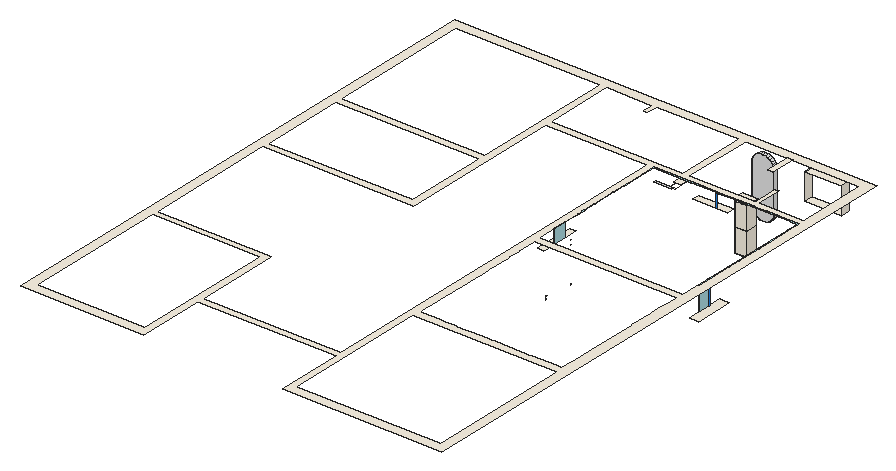
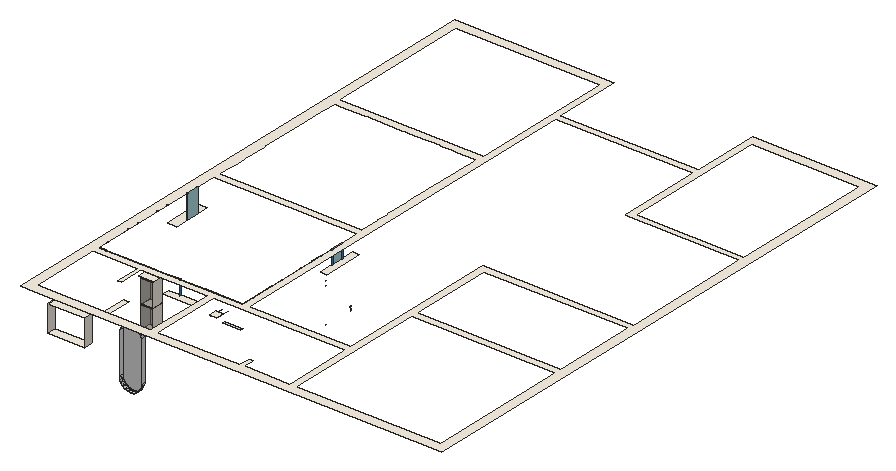
# SketchUp Ruby script. Lengths in inches.
U = 1.inch
M = Sketchup.active_model
def pt(a) = Geom::Point3d.new(a.map { |v| v * U })
def face(e, loops, mat)
  f = e.add_face(loops[0].map { |a| pt(a) })
  loops[1..].each { |l| e.add_face(l.map { |a| pt(a) }).erase! }
  f.material = f.back_material = mat if mat
  f
end
# faces: each face lists its corners as indices into pts; further lists are holes
def faces(e, pts, list, mat = nil) = list.each { |f| face(e, (f[0].is_a?(Array) ? f : [f]).map { |l| l.map { |i| pts[i] } }, mat) }
# xy, xz, yz: faces in a plane at the given z, y or x. An outline is a flat list of corners, or four numbers for a rectangle; further outlines are holes
def ring(l) = l.size == 4 ? [[l[0], l[1]], [l[2], l[1]], [l[2], l[3]], [l[0], l[3]]] : l.each_slice(2).to_a
def flat(e, list, mat, &to3) = list.each { |f| face(e, (f[0].is_a?(Array) ? f : [f]).map { |l| ring(l).map { |u, v| to3.(u, v) } }, mat) }
def xy(e, z, list, mat = nil) = flat(e, list, mat) { |x, y| [x, y, z] }
def xz(e, y, list, mat = nil) = flat(e, list, mat) { |x, z| [x, y, z] }
def yz(e, x, list, mat = nil) = flat(e, list, mat) { |y, z| [x, y, z] }
def lines(e, pts, list) = list.each { |a, b| e.add_line(pt(pts[a]), pt(pts[b])) }
# prism: a flat outline (further loops are holes) pulled along v
def prism(e, loops, v, mat = nil)
  f = face(e, loops, mat); d = Geom::Vector3d.new(v.map { |x| x * U })
  f.pushpull(f.normal.samedirection?(d) ? d.length : -d.length)
end
def box(e, o, s, mat = nil) = prism(e, [[o, [o[0] + s[0], o[1], o[2]], [o[0] + s[0], o[1] + s[1], o[2]], [o[0], o[1] + s[1], o[2]]]], [0, 0, s[2]], mat)
def at(x, y, z, deg = 0) = Geom::Transformation.translation(pt([x, y, z])) * Geom::Transformation.rotation(ORIGIN, Z_AXIS, deg.degrees)
def axes(o, x, y, z) = Geom::Transformation.new([*x, 0, *y, 0, *z, 0, *pt(o).to_a, 1])
def part(name) = M.definitions.add(name)
# library, detail: a bought-in or finely detailed component or shape, given as its bounding box
def library(name, o, s) = part(name).tap { |d| box(d.entities, o, s) }
def detail(e, o, s) = box(e.add_group.entities, o, s)
def put(e, d, t, mat = nil) = e.add_instance(d, t).tap { |i| i.material = mat if mat }
def group(e, t, mat = nil) = e.add_group.tap { |g| g.transformation = t; g.material = mat if mat }.entities
root = M.entities
M.materials.add("Material \#1").color = [140, 140, 140]
M.materials.add("[0030_OldLace]").color = [253, 245, 230]
M.materials.add("[0094_PowderBlue]").color = [176, 224, 230]
M.materials.add("[0098_DodgerBlue]").color = [30, 144, 255]
M.materials.add("[Mirror 02]").color = [229, 229, 229]
M.materials.add("[Translucent Glass Gray]").color = [128, 128, 128]
M.materials["[Translucent Glass Gray]"].alpha = 0.5
xy(root,58.602,[[264.049,358.92,264.049,358.939,264.045,358.932],[264.049,358.92,264.053,358.949,264.049,358.939],[264.049,358.92,264.054,358.932,264.053,358.949],[264.045,358.932,264.046,358.949,264.041,358.964],[264.045,358.932,264.049,358.939,264.046,358.949],
  [264.054,358.932,264.057,358.978,264.053,358.949],[264.054,358.932,264.058,358.964,264.057,358.978],[264.046,358.949,264.042,358.978,264.041,358.964],[264.041,358.964,264.042,358.978,264.038,359.014],[264.058,358.964,264.059,359.023,264.057,358.978],
  [264.058,358.964,264.061,359.014,264.059,359.023],[264.042,358.978,264.039,359.023,264.038,359.014],[264.038,359.014,264.039,359.023,264.037,359.075],[264.061,359.014,264.061,359.078,264.059,359.023],[264.061,359.014,264.062,359.075,264.061,359.078],
  [264.039,359.023,264.038,359.078,264.037,359.075],[264.037,359.075,264.038,359.078,264.037,359.14],[264.062,359.075,264.061,359.137,264.061,359.078],[264.062,359.075,264.062,359.14,264.061,359.137],[264.038,359.078,264.038,359.137,264.037,359.14],
  [264.038,359.137,264.038,359.201,264.037,359.14],[264.038,359.137,264.039,359.192,264.038,359.201],[264.061,359.137,264.062,359.14,264.059,359.192],[264.062,359.14,264.061,359.201,264.059,359.192],[264.039,359.192,264.041,359.251,264.038,359.201],
  [264.039,359.192,264.042,359.237,264.041,359.251],[264.059,359.192,264.061,359.201,264.057,359.237],[264.061,359.201,264.058,359.251,264.057,359.237],[264.042,359.237,264.045,359.284,264.041,359.251],[264.042,359.237,264.046,359.266,264.045,359.284],
  [264.057,359.237,264.058,359.251,264.053,359.266],[264.058,359.251,264.054,359.284,264.053,359.266],[264.046,359.266,264.049,359.295,264.045,359.284],[264.046,359.266,264.049,359.276,264.049,359.295],[264.053,359.266,264.054,359.284,264.049,359.276],
  [264.049,359.276,264.054,359.284,264.049,359.295]],"Material \#1")
xy(root,58.622,[[264.049,358.92,264.045,358.932,264.046,358.949],[264.049,358.92,264.046,358.949,264.049,358.939],[264.049,358.92,264.049,358.939,264.054,358.932],[264.045,358.932,264.041,358.964,264.042,358.978],[264.045,358.932,264.042,358.978,264.046,358.949],
  [264.054,358.932,264.049,358.939,264.053,358.949],[264.054,358.932,264.053,358.949,264.058,358.964],[264.053,358.949,264.057,358.978,264.058,358.964],[264.041,358.964,264.038,359.014,264.039,359.023],[264.041,358.964,264.039,359.023,264.042,358.978],
  [264.058,358.964,264.057,358.978,264.061,359.014],[264.057,358.978,264.059,359.023,264.061,359.014],[264.038,359.014,264.037,359.075,264.038,359.078],[264.038,359.014,264.038,359.078,264.039,359.023],[264.061,359.014,264.059,359.023,264.062,359.075],
  [264.059,359.023,264.061,359.078,264.062,359.075],[264.037,359.075,264.037,359.14,264.038,359.137],[264.037,359.075,264.038,359.137,264.038,359.078],[264.062,359.075,264.061,359.078,264.062,359.14],[264.061,359.078,264.061,359.137,264.062,359.14],
  [264.038,359.137,264.037,359.14,264.039,359.192],[264.061,359.137,264.059,359.192,264.061,359.201],[264.061,359.137,264.061,359.201,264.062,359.14],[264.037,359.14,264.038,359.201,264.039,359.192],[264.039,359.192,264.038,359.201,264.042,359.237],
  [264.059,359.192,264.057,359.237,264.058,359.251],[264.059,359.192,264.058,359.251,264.061,359.201],[264.038,359.201,264.041,359.251,264.042,359.237],[264.042,359.237,264.041,359.251,264.046,359.266],[264.057,359.237,264.053,359.266,264.054,359.284],
  [264.057,359.237,264.054,359.284,264.058,359.251],[264.041,359.251,264.045,359.284,264.046,359.266],[264.046,359.266,264.045,359.284,264.049,359.276],[264.053,359.266,264.049,359.276,264.049,359.295],[264.053,359.266,264.049,359.295,264.054,359.284],
  [264.049,359.276,264.045,359.284,264.049,359.295]],"Material \#1")
xy(root,70.574,[[346.166,460.902,357.778,472.402]],"[0030_OldLace]")
xy(root,71.074,[[346.166,460.902,357.778,472.402]],"[0030_OldLace]")
xy(root,87.625,[[356.125,535.465,392.375,544.465]],"[0030_OldLace]")
xy(root,93.657,[[346.166,460.902,357.778,472.402]],"[0030_OldLace]")
xy(root,93.765,[[264.049,358.92,264.046,358.949,264.045,358.932],[264.049,358.92,264.049,358.939,264.046,358.949],[264.049,358.92,264.054,358.932,264.049,358.939],[264.045,358.932,264.042,358.978,264.041,358.964],[264.045,358.932,264.046,358.949,264.042,358.978],
  [264.054,358.932,264.053,358.949,264.049,358.939],[264.054,358.932,264.058,358.964,264.053,358.949],[264.053,358.949,264.058,358.964,264.057,358.978],[264.041,358.964,264.039,359.023,264.038,359.014],[264.041,358.964,264.042,358.978,264.039,359.023],
  [264.058,358.964,264.061,359.014,264.057,358.978],[264.057,358.978,264.061,359.014,264.059,359.023],[264.038,359.014,264.038,359.078,264.037,359.075],[264.038,359.014,264.039,359.023,264.038,359.078],[264.061,359.014,264.062,359.075,264.059,359.023],
  [264.059,359.023,264.062,359.075,264.061,359.078],[264.037,359.075,264.038,359.078,264.038,359.137],[264.037,359.075,264.038,359.137,264.037,359.14],[264.062,359.075,264.062,359.14,264.061,359.078],[264.061,359.078,264.062,359.14,264.061,359.137],
  [264.038,359.137,264.039,359.192,264.037,359.14],[264.061,359.137,264.061,359.201,264.059,359.192],[264.061,359.137,264.062,359.14,264.061,359.201],[264.037,359.14,264.039,359.192,264.038,359.201],[264.039,359.192,264.042,359.237,264.038,359.201],
  [264.059,359.192,264.058,359.251,264.057,359.237],[264.059,359.192,264.061,359.201,264.058,359.251],[264.038,359.201,264.042,359.237,264.041,359.251],[264.042,359.237,264.046,359.266,264.041,359.251],[264.057,359.237,264.054,359.284,264.053,359.266],
  [264.057,359.237,264.058,359.251,264.054,359.284],[264.041,359.251,264.046,359.266,264.045,359.284],[264.046,359.266,264.049,359.276,264.045,359.284],[264.053,359.266,264.049,359.295,264.049,359.276],[264.053,359.266,264.054,359.284,264.049,359.295],
  [264.049,359.276,264.049,359.295,264.045,359.284]],"Material \#1")
xy(root,93.785,[[264.049,358.92,264.045,358.932,264.049,358.939],[264.049,358.92,264.049,358.939,264.053,358.949],[264.049,358.92,264.053,358.949,264.054,358.932],[264.045,358.932,264.041,358.964,264.046,358.949],[264.045,358.932,264.046,358.949,264.049,358.939],
  [264.054,358.932,264.053,358.949,264.057,358.978],[264.054,358.932,264.057,358.978,264.058,358.964],[264.046,358.949,264.041,358.964,264.042,358.978],[264.041,358.964,264.038,359.014,264.042,358.978],[264.058,358.964,264.057,358.978,264.059,359.023],
  [264.058,358.964,264.059,359.023,264.061,359.014],[264.042,358.978,264.038,359.014,264.039,359.023],[264.038,359.014,264.037,359.075,264.039,359.023],[264.061,359.014,264.059,359.023,264.061,359.078],[264.061,359.014,264.061,359.078,264.062,359.075],
  [264.039,359.023,264.037,359.075,264.038,359.078],[264.037,359.075,264.037,359.14,264.038,359.078],[264.062,359.075,264.061,359.078,264.061,359.137],[264.062,359.075,264.061,359.137,264.062,359.14],[264.038,359.078,264.037,359.14,264.038,359.137],
  [264.038,359.137,264.037,359.14,264.038,359.201],[264.038,359.137,264.038,359.201,264.039,359.192],[264.061,359.137,264.059,359.192,264.062,359.14],[264.062,359.14,264.059,359.192,264.061,359.201],[264.039,359.192,264.038,359.201,264.041,359.251],
  [264.039,359.192,264.041,359.251,264.042,359.237],[264.059,359.192,264.057,359.237,264.061,359.201],[264.061,359.201,264.057,359.237,264.058,359.251],[264.042,359.237,264.041,359.251,264.045,359.284],[264.042,359.237,264.045,359.284,264.046,359.266],
  [264.057,359.237,264.053,359.266,264.058,359.251],[264.058,359.251,264.053,359.266,264.054,359.284],[264.046,359.266,264.045,359.284,264.049,359.295],[264.046,359.266,264.049,359.295,264.049,359.276],[264.053,359.266,264.049,359.276,264.054,359.284],
  [264.049,359.276,264.049,359.295,264.054,359.284]],"Material \#1")
xy(root,94.157,[[346.166,460.902,357.778,472.402]],"[0030_OldLace]")
xy(root,96,[[410.75,323.465,410.75,334.965,411,334.965,411,335.465,410.75,335.465,410.75,347.465,411,347.465,411,347.965,410.75,347.965,410.75,361.527,420,361.527,420,323.465]],"[0030_OldLace]")
xy(root,98.228,[[264.049,358.92,264.049,358.939,264.045,358.932],[264.049,358.92,264.053,358.949,264.049,358.939],[264.049,358.92,264.054,358.932,264.053,358.949],[264.045,358.932,264.046,358.949,264.041,358.964],[264.045,358.932,264.049,358.939,264.046,358.949],
  [264.054,358.932,264.057,358.978,264.053,358.949],[264.054,358.932,264.058,358.964,264.057,358.978],[264.046,358.949,264.042,358.978,264.041,358.964],[264.041,358.964,264.042,358.978,264.038,359.014],[264.058,358.964,264.059,359.023,264.057,358.978],
  [264.058,358.964,264.061,359.014,264.059,359.023],[264.042,358.978,264.039,359.023,264.038,359.014],[264.038,359.014,264.039,359.023,264.037,359.075],[264.061,359.014,264.061,359.078,264.059,359.023],[264.061,359.014,264.062,359.075,264.061,359.078],
  [264.039,359.023,264.038,359.078,264.037,359.075],[264.037,359.075,264.038,359.078,264.037,359.14],[264.062,359.075,264.061,359.137,264.061,359.078],[264.062,359.075,264.062,359.14,264.061,359.137],[264.038,359.078,264.038,359.137,264.037,359.14],
  [264.038,359.137,264.038,359.201,264.037,359.14],[264.038,359.137,264.039,359.192,264.038,359.201],[264.061,359.137,264.062,359.14,264.059,359.192],[264.062,359.14,264.061,359.201,264.059,359.192],[264.039,359.192,264.041,359.251,264.038,359.201],
  [264.039,359.192,264.042,359.237,264.041,359.251],[264.059,359.192,264.061,359.201,264.057,359.237],[264.061,359.201,264.058,359.251,264.057,359.237],[264.042,359.237,264.045,359.284,264.041,359.251],[264.042,359.237,264.046,359.266,264.045,359.284],
  [264.057,359.237,264.058,359.251,264.053,359.266],[264.058,359.251,264.054,359.284,264.053,359.266],[264.046,359.266,264.049,359.295,264.045,359.284],[264.046,359.266,264.049,359.276,264.049,359.295],[264.053,359.266,264.054,359.284,264.049,359.276],
  [264.049,359.276,264.054,359.284,264.049,359.295]],"Material \#1")
xy(root,98.248,[[264.049,358.92,264.045,358.932,264.046,358.949],[264.049,358.92,264.046,358.949,264.049,358.939],[264.049,358.92,264.049,358.939,264.054,358.932],[264.045,358.932,264.041,358.964,264.042,358.978],[264.045,358.932,264.042,358.978,264.046,358.949],
  [264.054,358.932,264.049,358.939,264.053,358.949],[264.054,358.932,264.053,358.949,264.058,358.964],[264.053,358.949,264.057,358.978,264.058,358.964],[264.041,358.964,264.038,359.014,264.039,359.023],[264.041,358.964,264.039,359.023,264.042,358.978],
  [264.058,358.964,264.057,358.978,264.061,359.014],[264.057,358.978,264.059,359.023,264.061,359.014],[264.038,359.014,264.037,359.075,264.038,359.078],[264.038,359.014,264.038,359.078,264.039,359.023],[264.061,359.014,264.059,359.023,264.062,359.075],
  [264.059,359.023,264.061,359.078,264.062,359.075],[264.037,359.075,264.037,359.14,264.038,359.137],[264.037,359.075,264.038,359.137,264.038,359.078],[264.062,359.075,264.061,359.078,264.062,359.14],[264.061,359.078,264.061,359.137,264.062,359.14],
  [264.038,359.137,264.037,359.14,264.039,359.192],[264.061,359.137,264.059,359.192,264.061,359.201],[264.061,359.137,264.061,359.201,264.062,359.14],[264.037,359.14,264.038,359.201,264.039,359.192],[264.039,359.192,264.038,359.201,264.042,359.237],
  [264.059,359.192,264.057,359.237,264.058,359.251],[264.059,359.192,264.058,359.251,264.061,359.201],[264.038,359.201,264.041,359.251,264.042,359.237],[264.042,359.237,264.041,359.251,264.046,359.266],[264.057,359.237,264.053,359.266,264.054,359.284],
  [264.057,359.237,264.054,359.284,264.058,359.251],[264.041,359.251,264.045,359.284,264.046,359.266],[264.046,359.266,264.045,359.284,264.049,359.276],[264.053,359.266,264.049,359.276,264.049,359.295],[264.053,359.266,264.049,359.295,264.054,359.284],
  [264.049,359.276,264.045,359.284,264.049,359.295]],"Material \#1")
xy(root,102.757,[[262.134,465.465,279.821,468.027]],"[Mirror 02]")
xy(root,106,[[261,321.882,261,361.777,267.4375,361.777,267.4375,347.965,267,347.965,267,347.465,267.4375,347.465,267.4375,335.465,267,335.465,267,334.965,267.4375,334.965,267.4375,321.882],[306.3125,458.34,306.3125,465.465,341.0625,465.465,341.0625,458.34,329.5,458.34,329.5,459.465,329,459.465,329,458.34]],"[0030_OldLace]")
xy(root,109.284,[[281.161,465.465,288.974,472.965]],"[0030_OldLace]")
xy(root,114.125,[[356.125,535.465,392.375,544.465]],"[0030_OldLace]")
xy(root,117.24,[[346.166,460.902,357.778,472.402]],"[0030_OldLace]")
xy(root,119.066,[[344.34,465.465,359.604,472.402]],"[0030_OldLace]")
xy(root,120,[[[0,4.465,123,4.465,123,71.465,261,71.465,261,4.465,420,4.465,420,544.465,411,544.465,411,465.465,366.13,465.465,366.13,489.902,362.99,489.902,362.99,465.465,297,465.465,297,535.465,411,535.465,411,544.465,0,544.465],[123,77.465,123,162.902,9,162.902,9,295.465,159,295.465,159,459.465,261,459.465,261,77.465],[267,13.465,411,159.465],[410.75,315.215,410.75,315.465,267,315.465,267,459.465,411,459.465,411,315.215],[9,391.465,153,535.465],[291.481,165.465,291.481,166.152,267.8125,166.152,267.8125,178.468,267,178.468,267,178.961,268.125,178.961,268.125,202.965,267,202.965,267,203.457,268.125,203.457,268.125,215.465,267,215.465,267,215.965,268.125,215.965,268.125,239.965,267,239.965,267,240.465,268.125,240.465,268.125,252.527,267,252.527,267,252.996,268.125,252.996,268.125,276.965,267,276.965,267,277.465,268.125,277.465,268.125,289.465,267,289.465,267,289.965,268.125,289.965,268.125,307.965,267,307.965,267,309.465,410,309.465,410,289.965,411,289.965,411,289.465,410,289.465,410,277.469,411,277.469,411,276.965,410,276.965,410,252.965,411,252.965,411,252.474,410,252.474,410,240.465,411,240.465,411,239.968,410,239.968,410,215.965,411,215.965,411,215.463,410,215.463,410,203.465,411,203.465,411,202.965,410,202.965,410,179.003,411,179.003,411,178.44,410,178.44,410,166.152,403,166.152,403,165.465,402.494,165.465,402.494,166.152,378.5,166.152,378.5,165.465,378.006,165.465,378.006,166.152,366,166.152,366,165.465,365.494,165.465,365.494,166.152,341.448,166.152,341.448,165.465,340.998,165.465,340.998,166.152,329,166.152,329,165.465,328.501,165.465,328.501,166.152,304.5,166.152,304.5,165.465,304.001,165.465,304.001,166.152,292.007,166.152,292.007,165.465],[9,13.465,117,157.465],[9,301.465,153,385.465],[159,465.465,159,535.465,204.963,535.465,204.963,524.215,208.558,524.215,208.558,535.465,291,535.465,291,465.465]],[339.125,511.152,343.94,535.465]],"[0030_OldLace]")
xy(root,120,[[267,335.465,267.4375,347.465],[410.75,335.465,411,347.465],[267,347.965,267.4375,371.959],[410.75,347.965,411,371.965],[410.75,372.465,411,384.458],
  [267,372.47,267.4375,384.441],[267,384.939,267.4375,408.963],[410.75,384.961,411,408.962],[410.75,409.463,411,421.465],[267,409.486,267.4375,421.465],
  [267,421.965,267.4375,445.965],[410.75,421.965,411,445.965],[267,446.465,267.4375,446.465,267.4375,458.34,292,458.34,292,459.465,267,459.465],[410.75,446.465,411,446.465,411,459.465,403.488,459.465,403.488,458.34,410.75,458.34],[292.512,458.34,304.5,459.465],
  [305,458.34,329,459.465],[329.5,458.34,341.5,459.465],[342.008,458.34,366,459.465],[366.5,458.34,378.5,459.465],[379.002,458.34,402.988,459.465]],"[0094_PowderBlue]")
xz(root,328.199,[[263.949,58.441,263.973,58.441,263.949,58.476],[263.973,58.441,263.973,58.476,263.949,58.476],[264.08,58.441,264.104,58.441,264.104,58.476],[264.08,58.441,264.104,58.476,264.08,58.476]],"Material \#1")
xz(root,328.205,[[263.973,58.273,263.973,58.337,263.949,58.337],[264.08,58.273,264.104,58.337,264.08,58.337]],"Material \#1")
xz(root,328.207,[[263.949,58.385,263.973,58.385,263.949,58.413],[263.973,58.385,263.973,58.413,263.949,58.413],[264.08,58.385,264.104,58.385,264.104,58.413],[264.08,58.385,264.104,58.413,264.08,58.413]],"Material \#1")
xz(root,334.965,[[410.75,96,411,120],[267,106,267.4375,120]],"[0098_DodgerBlue]")
xz(root,335.465,[[410.75,96,411,120],[267,106,267.4375,120]],"[0098_DodgerBlue]")
xz(root,347.465,[[410.75,96,411,120],[267,106,267.4375,120]],"[0098_DodgerBlue]")
xz(root,347.965,[[410.75,96,411,120],[267,106,267.4375,120]],"[0098_DodgerBlue]")
xz(root,459.465,[[329,106,329.5,120]],"[0098_DodgerBlue]")
xz(root,460.902,[[346.166,71.074,357.778,93.657],[346.166,94.157,357.778,117.24]],"[0030_OldLace]")
xz(root,472.402,[[346.166,70.574,357.778,71.074],[346.166,93.657,357.778,94.157]],"[0030_OldLace]")
xz(root,472.402,[[346.166,71.074,357.778,93.657],[346.166,94.157,357.778,117.24]],"[Translucent Glass Gray]")
xz(root,531.882,[[317.334,57.921,320.182,58.264,322.836,59.27,325.115,60.869,326.864,62.954,327.964,65.381,328.339,67.986,328.339,109.181,327.518,111.378,326.18,113.35,324.394,114.999,322.25,116.241,319.856,117.012,317.334,117.273,314.812,117.012,312.418,116.241,310.273,114.999,308.487,113.35,307.149,111.378,306.328,109.181,306.328,67.986,306.703,65.381,307.803,62.954,309.552,60.869,311.831,59.27,314.485,58.264]],"[Mirror 02]")
yz(root,263.952,[[328.822,61.352,328.811,61.512,328.822,61.514],[328.811,61.512,328.781,61.656,328.792,61.661],[328.811,61.512,328.792,61.661,328.822,61.514],[328.781,61.656,328.743,61.796,328.792,61.661]],"Material \#1")
yz(root,263.975,[[328.177,58.05,328.229,58.097,328.177,58.089],[328.177,58.05,328.236,58.059,328.289,58.084],[328.177,58.05,328.276,58.12,328.229,58.097],[328.177,58.05,328.289,58.084,328.376,58.176],[328.177,58.05,328.376,58.176,328.276,58.12],
  [328.289,58.084,328.337,58.124,328.376,58.176],[328.276,58.12,328.376,58.176,328.318,58.155],[328.318,58.155,328.376,58.176,328.353,58.201],[328.376,58.176,328.379,58.256,328.353,58.201],[328.376,58.176,328.396,58.319,328.379,58.256],
  [328.376,58.176,328.406,58.239,328.425,58.31],[328.376,58.176,328.425,58.31,328.43,58.431],[328.376,58.176,328.43,58.431,328.396,58.319],[328.425,58.31,328.432,58.387,328.43,58.431],[328.396,58.319,328.43,58.431,328.402,58.387],
  [328.402,58.387,328.43,58.431,328.396,58.455],[328.43,58.431,328.325,58.666,328.353,58.572],[328.43,58.431,328.329,58.66,328.325,58.666],[328.43,58.431,328.333,58.654,328.329,58.66],[328.43,58.431,328.381,58.587,328.333,58.654],
  [328.43,58.431,328.353,58.572,328.379,58.517],[328.43,58.431,328.379,58.517,328.396,58.455],[328.43,58.431,328.412,58.514,328.381,58.587],[328.43,58.431,328.423,58.474,328.412,58.514],[328.412,58.514,328.398,58.552,328.381,58.587],
  [328.353,58.572,328.325,58.666,328.318,58.619],[328.381,58.587,328.337,58.648,328.333,58.654],[328.381,58.587,328.36,58.619,328.337,58.648],[328.318,58.619,328.325,58.666,328.276,58.654],[328.276,58.654,328.325,58.666,328.229,58.676],
  [328.325,58.666,328.321,58.679,328.229,58.676],[328.325,58.666,328.323,58.672,328.321,58.679],[328.029,58.667,328.32,59.055,328.316,59.098],[328.126,58.676,328.177,58.684,328.32,59.055],[328.229,58.676,328.32,59.055,328.177,58.684],
  [328.229,58.676,328.32,58.695,328.32,59.055],[328.229,58.676,328.321,58.679,328.32,58.695],[328.321,58.679,328.32,58.687,328.32,58.695],[328.316,59.098,328.24,59.224,328.115,59.224],[328.316,59.098,328.288,59.173,328.24,59.224],
  [328.316,59.098,328.305,59.138,328.288,59.173],[328.288,59.173,328.266,59.202,328.24,59.224],[328.24,59.224,328.21,59.239,328.177,59.244]],"Material \#1")
yz(root,264.078,[[328.177,58.05,328.177,58.089,328.229,58.097],[328.177,58.05,328.229,58.097,328.276,58.12],[328.177,58.05,328.276,58.12,328.376,58.176],[328.177,58.05,328.289,58.084,328.236,58.059],[328.177,58.05,328.376,58.176,328.289,58.084],
  [328.289,58.084,328.376,58.176,328.337,58.124],[328.276,58.12,328.318,58.155,328.376,58.176],[328.318,58.155,328.353,58.201,328.376,58.176],[328.376,58.176,328.353,58.201,328.379,58.256],[328.376,58.176,328.379,58.256,328.396,58.319],
  [328.376,58.176,328.396,58.319,328.43,58.431],[328.376,58.176,328.425,58.31,328.406,58.239],[328.376,58.176,328.43,58.431,328.425,58.31],[328.425,58.31,328.43,58.431,328.432,58.387],[328.396,58.319,328.402,58.387,328.43,58.431],
  [328.402,58.387,328.396,58.455,328.43,58.431],[328.43,58.431,328.325,58.666,328.329,58.66],[328.43,58.431,328.353,58.572,328.325,58.666],[328.43,58.431,328.329,58.66,328.333,58.654],[328.43,58.431,328.333,58.654,328.381,58.587],
  [328.43,58.431,328.379,58.517,328.353,58.572],[328.43,58.431,328.396,58.455,328.379,58.517],[328.43,58.431,328.381,58.587,328.412,58.514],[328.43,58.431,328.412,58.514,328.423,58.474],[328.412,58.514,328.381,58.587,328.398,58.552],
  [328.353,58.572,328.318,58.619,328.325,58.666],[328.381,58.587,328.333,58.654,328.337,58.648],[328.381,58.587,328.337,58.648,328.36,58.619],[328.318,58.619,328.276,58.654,328.325,58.666],[328.276,58.654,328.229,58.676,328.325,58.666],
  [328.325,58.666,328.229,58.676,328.321,58.679],[328.325,58.666,328.321,58.679,328.323,58.672],[328.029,58.667,328.316,59.098,328.32,59.055],[328.126,58.676,328.32,59.055,328.177,58.684],[328.229,58.676,328.177,58.684,328.32,59.055],
  [328.229,58.676,328.32,58.695,328.321,58.679],[328.229,58.676,328.32,59.055,328.32,58.695],[328.321,58.679,328.32,58.695,328.32,58.687],[328.316,59.098,328.115,59.224,328.24,59.224],[328.316,59.098,328.24,59.224,328.288,59.173],
  [328.316,59.098,328.288,59.173,328.305,59.138],[328.288,59.173,328.24,59.224,328.266,59.202],[328.24,59.224,328.177,59.244,328.21,59.239]],"Material \#1")
yz(root,264.101,[[328.822,61.352,328.822,61.514,328.811,61.512],[328.822,61.352,328.833,61.353,328.822,61.514],[328.216,61.422,328.214,61.437,328.177,61.432],[328.216,61.422,328.253,61.436,328.214,61.437],[328.253,61.436,328.249,61.45,328.214,61.437],
  [328.253,61.436,328.287,61.457,328.249,61.45],[328.249,61.45,328.287,61.457,328.281,61.47],[328.287,61.457,328.318,61.485,328.281,61.47],[328.281,61.47,328.318,61.485,328.31,61.497],[328.318,61.485,328.344,61.52,328.31,61.497],
  [328.31,61.497,328.344,61.52,328.335,61.53],[328.811,61.512,328.792,61.661,328.781,61.656],[328.811,61.512,328.822,61.514,328.792,61.661],[328.344,61.52,328.365,61.56,328.335,61.53],[328.335,61.53,328.365,61.56,328.355,61.568],
  [328.365,61.56,328.381,61.605,328.355,61.568],[328.355,61.568,328.381,61.605,328.371,61.61],[328.381,61.605,328.392,61.654,328.371,61.61],[328.371,61.61,328.392,61.654,328.38,61.657],[328.392,61.654,328.395,61.705,328.38,61.657],
  [328.781,61.656,328.743,61.796,328.734,61.788],[328.781,61.656,328.792,61.661,328.743,61.796],[328.38,61.657,328.395,61.705,328.384,61.705],[328.384,61.705,328.392,61.757,328.38,61.754],[328.384,61.705,328.395,61.705,328.392,61.757],
  [328.38,61.754,328.381,61.806,328.371,61.8],[328.38,61.754,328.392,61.757,328.381,61.806],[328.734,61.788,328.679,61.917,328.67,61.907],[328.734,61.788,328.743,61.796,328.679,61.917],[328.371,61.8,328.365,61.851,328.355,61.843],
  [328.371,61.8,328.381,61.806,328.365,61.851],[328.355,61.843,328.344,61.891,328.335,61.881],[328.355,61.843,328.365,61.851,328.344,61.891],[328.335,61.881,328.318,61.925,328.31,61.914],[328.335,61.881,328.344,61.891,328.318,61.925],
  [328.67,61.907,328.6,62.021,328.592,62.01],[328.67,61.907,328.679,61.917,328.6,62.021],[328.31,61.914,328.287,61.954,328.281,61.941],[328.31,61.914,328.318,61.925,328.287,61.954],[328.281,61.941,328.253,61.975,328.249,61.961],
  [328.281,61.941,328.287,61.954,328.253,61.975],[328.249,61.961,328.216,61.989,328.214,61.974],[328.249,61.961,328.253,61.975,328.216,61.989],[328.214,61.974,328.216,61.989,328.177,61.993],[328.592,62.01,328.508,62.107,328.502,62.094],
  [328.592,62.01,328.6,62.021,328.508,62.107],[328.502,62.094,328.406,62.171,328.402,62.157],[328.502,62.094,328.508,62.107,328.406,62.171],[328.402,62.157,328.295,62.211,328.293,62.196],[328.402,62.157,328.406,62.171,328.295,62.211],
  [328.293,62.196,328.177,62.225,328.177,62.21],[328.293,62.196,328.295,62.211,328.177,62.225]],"Material \#1")
yz(root,264.103,[[328.177,58.05,328.229,58.097,328.177,58.089],[328.177,58.05,328.236,58.059,328.289,58.084],[328.177,58.05,328.276,58.12,328.229,58.097],[328.177,58.05,328.289,58.084,328.376,58.176],[328.177,58.05,328.376,58.176,328.276,58.12],
  [328.289,58.084,328.337,58.124,328.376,58.176],[328.276,58.12,328.376,58.176,328.318,58.155],[328.318,58.155,328.376,58.176,328.353,58.201],[328.376,58.176,328.379,58.256,328.353,58.201],[328.376,58.176,328.406,58.239,328.425,58.31],
  [328.376,58.176,328.425,58.31,328.43,58.431],[328.376,58.176,328.43,58.431,328.379,58.256],[328.379,58.256,328.43,58.431,328.396,58.319],[328.425,58.31,328.432,58.387,328.43,58.431],[328.396,58.319,328.43,58.431,328.402,58.387],
  [328.402,58.387,328.43,58.431,328.396,58.455],[328.43,58.431,328.325,58.666,328.379,58.517],[328.43,58.431,328.329,58.66,328.325,58.666],[328.43,58.431,328.333,58.654,328.329,58.66],[328.43,58.431,328.381,58.587,328.333,58.654],
  [328.43,58.431,328.379,58.517,328.396,58.455],[328.43,58.431,328.412,58.514,328.381,58.587],[328.43,58.431,328.423,58.474,328.412,58.514],[328.412,58.514,328.398,58.552,328.381,58.587],[328.379,58.517,328.325,58.666,328.353,58.572],
  [328.002,58.572,328.037,58.619,328.288,59.173],[328.353,58.572,328.321,58.679,328.318,58.619],[328.353,58.572,328.325,58.666,328.321,58.679],[328.381,58.587,328.337,58.648,328.333,58.654],[328.381,58.587,328.36,58.619,328.337,58.648],
  [328.037,58.619,328.078,58.654,328.288,59.173],[328.318,58.619,328.32,59.055,328.276,58.654],[328.318,58.619,328.32,58.695,328.32,59.055],[328.318,58.619,328.321,58.679,328.32,58.695],[328.276,58.654,328.32,59.055,328.229,58.676],
  [328.325,58.666,328.323,58.672,328.321,58.679],[328.029,58.667,328.288,59.173,328.032,58.673],[328.032,58.673,328.288,59.173,328.033,58.68],[328.126,58.676,328.177,58.684,328.288,59.173],[328.229,58.676,328.32,59.055,328.177,58.684],
  [328.321,58.679,328.32,58.687,328.32,58.695],[328.033,58.68,328.288,59.173,328.034,58.6875],[328.177,58.684,328.32,59.055,328.288,59.173],[328.32,59.055,328.316,59.098,328.288,59.173],[328.316,59.098,328.305,59.138,328.288,59.173],
  [328.288,59.173,328.24,59.224,328.177,59.244],[328.288,59.173,328.266,59.202,328.24,59.224],[328.24,59.224,328.21,59.239,328.177,59.244]],"Material \#1")
yz(root,267,[[334.965,106,335.465,120],[347.465,106,347.965,120]],"[0098_DodgerBlue]")
yz(root,267.4375,[[335.465,106,347.465,120]],"[0094_PowderBlue]")
yz(root,306.328,[[531.882,67.986,535.465,109.181]],"[Mirror 02]")
yz(root,328.339,[[531.882,67.986,535.465,109.181]],"[Mirror 02]")
yz(root,329,[[458.34,106,459.465,120]],"[0098_DodgerBlue]")
yz(root,329.5,[[458.34,106,459.465,120]],"[0098_DodgerBlue]")
yz(root,346.166,[[460.902,70.574,472.402,71.074],[460.902,71.074,472.402,93.657],[460.902,93.657,472.402,94.157],[460.902,94.157,472.402,117.24]],"[0030_OldLace]")
yz(root,356.125,[[535.465,87.625,544.465,114.125]],"[0030_OldLace]")
yz(root,357.778,[[460.902,71.074,472.402,93.657],[460.902,94.157,472.402,117.24]],"[0030_OldLace]")
yz(root,392.375,[[535.465,87.625,544.465,114.125]],"[0030_OldLace]")
yz(root,410.75,[[335.465,96,347.465,120]],"[0094_PowderBlue]")
yz(root,411,[[334.965,96,335.465,120],[347.465,96,347.965,120]],"[0098_DodgerBlue]")
p = [[314.485,535.465,57.356],[317.334,535.465,56.981],[314.485,531.882,58.264],[317.334,531.882,57.921],[320.182,535.465,57.356],[311.831,535.465,58.455],
  [311.831,531.882,59.27],[320.182,531.882,58.264],[322.836,535.465,58.455],[263.949,328.202,58.261],[263.949,328.205,58.189],[263.973,328.205,58.189],
  [263.973,328.205,58.189],[263.973,328.205,58.253],[263.949,328.202,58.261],[264.104,328.202,58.261],[264.08,328.205,58.253],[264.08,328.205,58.189],
  [264.08,328.205,58.189],[264.104,328.205,58.189],[264.104,328.202,58.261],[263.949,328.205,58.337],[263.949,328.202,58.261],[263.973,328.205,58.273],
  [263.949,328.199,58.357],[263.949,328.205,58.337],[263.973,328.205,58.337],[263.973,328.205,58.337],[263.973,328.199,58.357],[263.949,328.199,58.357],
  [264.104,328.199,58.357],[264.08,328.199,58.357],[264.08,328.205,58.337],[264.08,328.205,58.337],[264.104,328.205,58.337],[264.104,328.199,58.357],
  [264.08,328.205,58.273],[264.104,328.202,58.261],[264.104,328.205,58.337],[322.836,531.882,59.27],[263.949,328.207,58.385],[263.949,328.199,58.357],
  [263.973,328.199,58.357],[263.949,328.199,58.441],[263.949,328.207,58.413],[263.973,328.207,58.413],[263.973,328.199,58.441],[263.973,328.199,58.357],
  [263.973,328.207,58.385],[263.949,328.207,58.385],[264.104,328.199,58.441],[264.08,328.199,58.441],[264.08,328.207,58.413],[264.104,328.207,58.385],
  [264.08,328.207,58.385],[264.08,328.199,58.357],[264.08,328.207,58.413],[264.104,328.207,58.413],[264.104,328.199,58.441],[264.08,328.199,58.357],
  [264.104,328.199,58.357],[264.104,328.207,58.385],[263.949,328.191,58.518],[263.949,328.199,58.476],[263.973,328.199,58.476],[263.949,328.191,58.55],
  [263.949,328.191,58.518],[263.973,328.194,58.523],[263.973,328.194,58.545],[263.973,328.199,58.476],[263.973,328.188,58.513],[263.949,328.191,58.518],
  [264.104,328.191,58.518],[264.08,328.188,58.513],[264.08,328.199,58.476],[264.104,328.191,58.55],[264.08,328.194,58.545],[264.08,328.194,58.523],
  [264.104,328.191,58.518],[264.08,328.199,58.476],[264.104,328.199,58.476],[264.104,328.191,58.518],[309.552,535.465,60.204],[309.552,531.882,60.869],
  [325.115,535.465,60.204],[263.949,328.199,58.585],[263.949,328.191,58.55],[263.973,328.188,58.555],[263.973,328.188,58.555],[263.973,328.199,58.585],
  [263.949,328.199,58.585],[264.104,328.199,58.585],[264.08,328.199,58.585],[264.08,328.188,58.555],[264.08,328.188,58.555],[264.104,328.191,58.55],
  [264.104,328.199,58.585],[325.115,531.882,60.869],[307.803,535.465,62.483],[326.864,531.882,62.954],[326.864,535.465,62.483],[307.803,531.882,62.954],
  [306.703,535.465,65.138],[327.964,531.882,65.381],[327.964,535.465,65.138],[306.703,531.882,65.381],[306.328,535.465,67.986],[328.339,535.465,67.986],
  [306.328,531.882,67.986],[328.339,531.882,67.986],[307.149,535.465,111.378],[306.328,535.465,109.181],[306.328,531.882,109.181],[307.149,531.882,111.378],
  [328.339,535.465,109.181],[327.518,535.465,111.378],[327.518,531.882,111.378],[328.339,531.882,109.181],[308.487,535.465,113.35],[308.487,531.882,113.35],
  [326.18,535.465,113.35],[326.18,531.882,113.35],[310.273,535.465,114.999],[310.273,531.882,114.999],[324.394,535.465,114.999],[324.394,531.882,114.999],
  [312.418,535.465,116.241],[312.418,531.882,116.241],[322.25,535.465,116.241],[322.25,531.882,116.241],[314.812,535.465,117.012],[314.812,531.882,117.012],
  [319.856,535.465,117.012],[319.856,531.882,117.012],[317.334,535.465,117.273],[317.334,531.882,117.273],[282.327,472.965,108.118],[282.327,458.34,108.118],
  [287.808,472.965,108.118],[287.808,458.34,108.118]]
faces(root,p,[[0,1,2],[3,2,1],[1,4,3],[5,0,6],[2,6,0],[7,3,4],[4,8,7],[39,7,8],
  [82,5,83],[6,83,5],[8,84,39],[97,39,84],[82,83,98],[97,84,99],[100,99,84],[101,98,83],
  [98,101,102],[99,100,103],[104,103,100],[105,102,101],[102,105,106],[104,107,103],[108,106,105],[109,103,107]],"[0030_OldLace]")
faces(root,p,[[9,10,11],[12,13,14],[15,16,17],[18,19,20],[21,22,23],[24,25,26],[27,28,29],[30,31,32],
  [33,34,35],[36,37,38],[40,41,42],[43,44,45],[45,46,43],[47,48,49],[50,51,52],[53,54,55],
  [56,57,58],[59,60,61],[62,63,64],[65,66,67],[67,68,65],[69,70,71],[72,73,74],[75,76,77],
  [77,78,75],[79,80,81],[85,86,87],[88,89,90],[91,92,93],[94,95,96]],"Material \#1")
faces(root,p,[[110,111,112,113],[114,115,116,117],[118,110,113,119],[115,120,121,116],[122,118,119,123],[120,124,125,121],[126,122,123,127],[124,128,129,125],
  [130,126,127,131],[128,132,133,129],[134,130,131,135],[132,134,135,133]],"[Mirror 02]")
lines(root,p,[[136,137],[138,139]])
